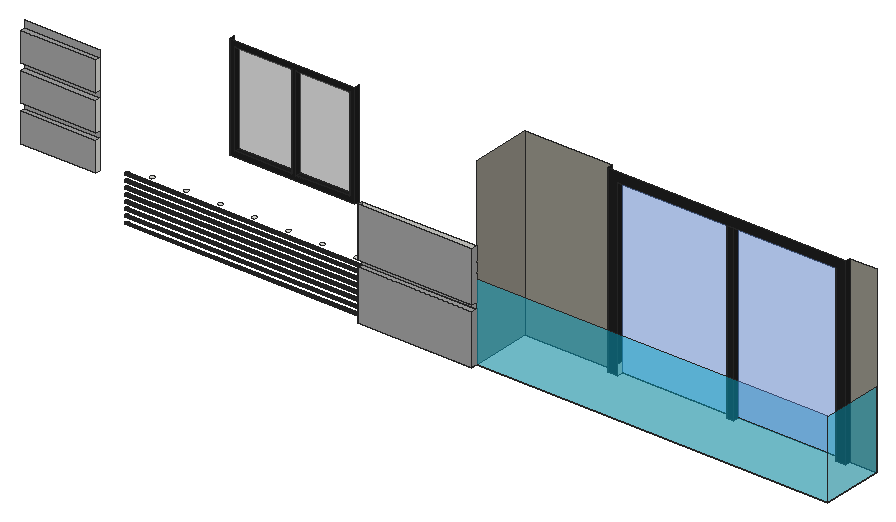
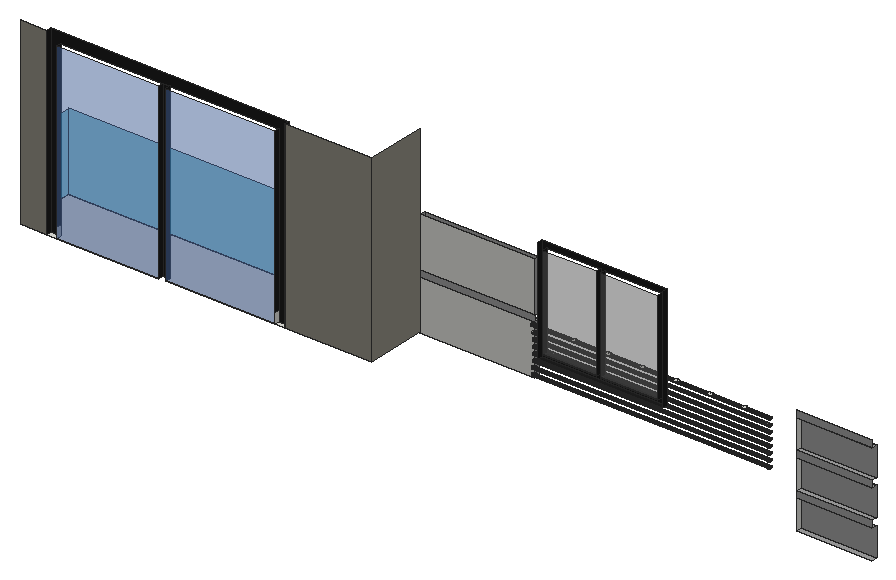
# SketchUp Ruby script. Lengths in inches.
U = 1.inch
M = Sketchup.active_model
def pt(a) = Geom::Point3d.new(a.map { |v| v * U })
def face(e, loops, mat)
  f = e.add_face(loops[0].map { |a| pt(a) })
  loops[1..].each { |l| e.add_face(l.map { |a| pt(a) }).erase! }
  f.material = f.back_material = mat if mat
  f
end
# faces: each face lists its corners as indices into pts; further lists are holes
def faces(e, pts, list, mat = nil) = list.each { |f| face(e, (f[0].is_a?(Array) ? f : [f]).map { |l| l.map { |i| pts[i] } }, mat) }
# xy, xz, yz: faces in a plane at the given z, y or x. An outline is a flat list of corners, or four numbers for a rectangle; further outlines are holes
def ring(l) = l.size == 4 ? [[l[0], l[1]], [l[2], l[1]], [l[2], l[3]], [l[0], l[3]]] : l.each_slice(2).to_a
def flat(e, list, mat, &to3) = list.each { |f| face(e, (f[0].is_a?(Array) ? f : [f]).map { |l| ring(l).map { |u, v| to3.(u, v) } }, mat) }
def xy(e, z, list, mat = nil) = flat(e, list, mat) { |x, y| [x, y, z] }
def xz(e, y, list, mat = nil) = flat(e, list, mat) { |x, z| [x, y, z] }
def yz(e, x, list, mat = nil) = flat(e, list, mat) { |y, z| [x, y, z] }
def lines(e, pts, list) = list.each { |a, b| e.add_line(pt(pts[a]), pt(pts[b])) }
# prism: a flat outline (further loops are holes) pulled along v
def prism(e, loops, v, mat = nil)
  f = face(e, loops, mat); d = Geom::Vector3d.new(v.map { |x| x * U })
  f.pushpull(f.normal.samedirection?(d) ? d.length : -d.length)
end
def box(e, o, s, mat = nil) = prism(e, [[o, [o[0] + s[0], o[1], o[2]], [o[0] + s[0], o[1] + s[1], o[2]], [o[0], o[1] + s[1], o[2]]]], [0, 0, s[2]], mat)
def at(x, y, z, deg = 0) = Geom::Transformation.translation(pt([x, y, z])) * Geom::Transformation.rotation(ORIGIN, Z_AXIS, deg.degrees)
def axes(o, x, y, z) = Geom::Transformation.new([*x, 0, *y, 0, *z, 0, *pt(o).to_a, 1])
def part(name) = M.definitions.add(name)
# library, detail: a bought-in or finely detailed component or shape, given as its bounding box
def library(name, o, s) = part(name).tap { |d| box(d.entities, o, s) }
def detail(e, o, s) = box(e.add_group.entities, o, s)
def put(e, d, t, mat = nil) = e.add_instance(d, t).tap { |i| i.material = mat if mat }
def group(e, t, mat = nil) = e.add_group.tap { |g| g.transformation = t; g.material = mat if mat }.entities
root = M.entities
M.materials.add("[0133_Gray]").color = [128, 128, 128]
M.materials.add("[Blacktop New]").color = [30, 30, 30]
M.materials.add("[Formica Graystone]").color = [149, 146, 135]
M.materials.add("[Marble Carrara Gold Floor Tile]").color = [225, 223, 217]
M.materials.add("[Pavers Flagstone Gray]").color = [162, 162, 162]
M.materials.add("[Translucent Glass Blue]").color = [100, 149, 237]
M.materials["[Translucent Glass Blue]"].alpha = 0.5
M.materials.add("[Translucent Glass Gray]").color = [128, 128, 128]
M.materials["[Translucent Glass Gray]"].alpha = 0.5
M.materials.add("[Translucent Glass Tinted]").color = [8, 201, 241]
M.materials["[Translucent Glass Tinted]"].alpha = 0.48
xy(root,368.26,[[0,36,45.0625,39]],"[Pavers Flagstone Gray]")
xy(root,369.12,[[229.62,0,297.58,3]],"[Pavers Flagstone Gray]")
xy(root,369.51,[[349.33,36,355.33,39],[484.79,36,490.79,39]])
xy(root,369.51,[[297.58,3,506.625,3,506.625,39,490.79,39,490.79,36,484.79,36,484.79,39,424.01,39,424.01,36,420.06,36,420.06,39,355.33,39,355.33,36,349.33,36,349.33,39,297.58,39]],"[Marble Carrara Gold Floor Tile]")
xy(root,385.625,[[0,36,45.0625,39]],"[Pavers Flagstone Gray]")
xy(root,389.7,[[0,36,45.0625,39]],"[Pavers Flagstone Gray]")
xy(root,399,[[229.62,0,297.58,3]],"[Pavers Flagstone Gray]")
xy(root,399.54,[[102.46,4.79,102.74,4.8,103.01,4.88,103.24,5.03,103.43,5.23,103.5625,5.48,103.625,5.75,103.61,6.02,103.53,6.29,103.39,6.52,103.18,6.71,102.94,6.84,102.67,6.91,102.39,6.9,102.13,6.82,101.89,6.67,101.7,6.47,101.57,6.22,101.51,5.95,101.52,5.68,101.6,5.41,101.75,5.17,101.95,4.99,102.19,4.85],[122.71,4.79,122.99,4.8,123.26,4.88,123.49,5.03,123.68,5.23,123.8125,5.48,123.875,5.75,123.86,6.02,123.78,6.29,123.64,6.52,123.43,6.71,123.19,6.84,122.92,6.91,122.64,6.9,122.38,6.82,122.14,6.67,121.95,6.47,121.82,6.22,121.76,5.95,121.77,5.68,121.85,5.41,122,5.17,122.2,4.99,122.44,4.85],[142.96,4.79,143.24,4.8,143.51,4.88,143.74,5.03,143.93,5.23,144.0625,5.48,144.125,5.75,144.11,6.02,144.03,6.29,143.89,6.52,143.68,6.71,143.44,6.84,143.17,6.91,142.89,6.9,142.63,6.82,142.39,6.67,142.2,6.47,142.07,6.22,142.01,5.95,142.02,5.68,142.1,5.41,142.25,5.17,142.45,4.99,142.69,4.85],[163.21,4.79,163.49,4.8,163.76,4.88,163.99,5.03,164.18,5.23,164.3125,5.48,164.375,5.75,164.36,6.02,164.28,6.29,164.14,6.52,163.93,6.71,163.69,6.84,163.42,6.91,163.14,6.9,162.88,6.82,162.64,6.67,162.45,6.47,162.32,6.22,162.26,5.95,162.27,5.68,162.35,5.41,162.5,5.17,162.7,4.99,162.94,4.85],[183.46,4.79,183.74,4.8,184.01,4.88,184.24,5.03,184.43,5.23,184.5625,5.48,184.625,5.75,184.61,6.02,184.53,6.29,184.39,6.52,184.18,6.71,183.94,6.84,183.67,6.91,183.39,6.9,183.13,6.82,182.89,6.67,182.7,6.47,182.57,6.22,182.51,5.95,182.52,5.68,182.6,5.41,182.75,5.17,182.95,4.99,183.19,4.85],
  [203.71,4.79,203.99,4.8,204.26,4.88,204.49,5.03,204.68,5.23,204.8125,5.48,204.875,5.75,204.86,6.02,204.78,6.29,204.64,6.52,204.43,6.71,204.19,6.84,203.92,6.91,203.64,6.9,203.38,6.82,203.14,6.67,202.95,6.47,202.82,6.22,202.76,5.95,202.77,5.68,202.85,5.41,203,5.17,203.2,4.99,203.44,4.85],[223.96,4.79,224.24,4.8,224.51,4.88,224.74,5.03,224.93,5.23,225.0625,5.48,225.125,5.75,225.11,6.02,225.03,6.29,224.89,6.52,224.68,6.71,224.44,6.84,224.17,6.91,223.89,6.9,223.63,6.82,223.39,6.67,223.2,6.47,223.07,6.22,223.01,5.95,223.02,5.68,223.1,5.41,223.25,5.17,223.45,4.99,223.69,4.85]])
xy(root,402.62,[[229.62,0,297.58,3]],"[Pavers Flagstone Gray]")
xy(root,405.86,[[124.42,36,198.67,39]],"[Blacktop New]")
xy(root,407.0625,[[0,36,45.0625,39]],"[Pavers Flagstone Gray]")
xy(root,408.86,[[127.42,36,161.55,39],[163.99,36,195.67,39]],"[Blacktop New]")
xy(root,411.14,[[0,36,45.0625,39]],"[Pavers Flagstone Gray]")
xy(root,428.5,[[0,36,45.0625,39]],"[Pavers Flagstone Gray]")
xz(root,0,[[229.62,369.12,297.58,399],[229.62,402.62,297.58,432.5]],"[Pavers Flagstone Gray]")
xz(root,3,[[229.62,369.12,297.58,399],[229.62,402.62,297.58,432.5]])
xz(root,3,[[229.62,399,297.58,402.62]],"[Pavers Flagstone Gray]")
xz(root,3,[[297.58,369.51,506.625,415.41]],"[Translucent Glass Tinted]")
xz(root,36,[[349.33,369.51,355.33,369.51,355.33,472.125,484.79,472.125,484.79,369.51,490.79,369.51,490.79,478.125,349.33,478.125],[420.06,369.51,424.01,472.125],[[124.42,405.86,198.67,467.74],[127.42,408.86,161.55,464.74],[163.99,408.86,195.67,464.74]]],"[Blacktop New]")
xz(root,36,[[0,368.26,45.0625,385.625],[0,389.7,45.0625,407.0625],[0,411.14,45.0625,428.5]],"[Pavers Flagstone Gray]")
xz(root,39,[[297.58,369.51,349.33,478.125],[490.79,369.51,506.625,478.125]],"[Formica Graystone]")
xz(root,39,[[0,385.625,45.0625,389.7],[0,407.0625,45.0625,411.14],[0,428.5,45.0625,432.57]],"[Pavers Flagstone Gray]")
xz(root,39,[[355.33,369.51,420.06,472.125],[424.01,369.51,484.79,472.125]],"[Translucent Glass Blue]")
xz(root,39,[[127.42,408.86,161.55,464.74],[163.99,408.86,195.67,464.74]],"[Translucent Glass Gray]")
yz(root,45.0625,[[36,368.26,39,385.625],[36,389.7,39,407.0625],[36,411.14,39,428.5]])
yz(root,124.42,[[36,405.86,39,467.74]],"[Blacktop New]")
yz(root,127.42,[[36,408.86,39,464.74]],"[Blacktop New]")
yz(root,161.55,[[36,408.86,39,464.74]],"[Blacktop New]")
yz(root,163.99,[[36,408.86,39,464.74]],"[Blacktop New]")
yz(root,195.67,[[36,408.86,39,464.74]],"[Blacktop New]")
yz(root,198.67,[[36,405.86,39,467.74]],"[Blacktop New]")
yz(root,229.62,[[0,369.12,3,399],[0,402.62,3,432.5]],"[Pavers Flagstone Gray]")
yz(root,229.85,[[3.75,393.11,3.93,393.13,4.1,393.2,4.24,393.31,4.35,393.45,4.42,393.61,4.44,393.79,4.42,393.97,4.35,394.14,4.24,394.28,4.1,394.39,3.93,394.46,3.75,394.48,3.57,394.46,3.41,394.39,3.27,394.28,3.16,394.14,3.09,393.97,3.06,393.79,3.09,393.61,3.16,393.45,3.27,393.31,3.41,393.2,3.57,393.13]])
yz(root,230.1,[[3.75,370.61,3.93,370.63,4.1,370.7,4.24,370.81,4.35,370.95,4.42,371.11,4.44,371.29,4.42,371.47,4.35,371.64,4.24,371.78,4.1,371.89,3.93,371.96,3.75,371.98,3.57,371.96,3.41,371.89,3.27,371.78,3.16,371.64,3.09,371.47,3.06,371.29,3.09,371.11,3.16,370.95,3.27,370.81,3.41,370.7,3.57,370.63]])
yz(root,230.16,[[3.75,374.36,3.93,374.38,4.1,374.45,4.24,374.56,4.35,374.7,4.42,374.86,4.44,375.04,4.42,375.22,4.35,375.39,4.24,375.53,4.1,375.64,3.93,375.71,3.75,375.73,3.57,375.71,3.41,375.64,3.27,375.53,3.16,375.39,3.09,375.22,3.06,375.04,3.09,374.86,3.16,374.7,3.27,374.56,3.41,374.45,3.57,374.38]])
yz(root,230.66,[[3.75,396.86,3.93,396.88,4.1,396.95,4.24,397.06,4.35,397.2,4.42,397.36,4.44,397.54,4.42,397.72,4.35,397.89,4.24,398.03,4.1,398.14,3.93,398.21,3.75,398.23,3.57,398.21,3.41,398.14,3.27,398.03,3.16,397.89,3.09,397.72,3.06,397.54,3.09,397.36,3.16,397.2,3.27,397.06,3.41,396.95,3.57,396.88]])
yz(root,297.58,[[0,369.12,3,369.51]])
yz(root,297.58,[[3,369.51,39,478.125]],"[Formica Graystone]")
yz(root,297.58,[[0,369.51,3,399],[0,402.62,3,432.5]],"[Pavers Flagstone Gray]")
yz(root,349.33,[[36,369.51,39,478.125]],"[Blacktop New]")
yz(root,355.33,[[36,369.51,39,375.51]])
yz(root,355.33,[[36,375.51,39,472.125]],"[Blacktop New]")
yz(root,420.06,[[36,369.51,39,472.125]],"[Blacktop New]")
yz(root,424.01,[[36,369.51,39,472.125]],"[Blacktop New]")
yz(root,484.79,[[36,369.51,39,375.51]])
yz(root,484.79,[[36,375.51,39,472.125]],"[Blacktop New]")
yz(root,490.79,[[36,369.51,39,478.125]],"[Blacktop New]")
yz(root,506.625,[[3,369.51,39,415.33]],"[Translucent Glass Tinted]")
p = [[88.53,3.41,370.7],[88.53,3.57,370.63],[230.1,3.57,370.63],[230.1,3.41,370.7],[88.53,3.75,370.61],[230.1,3.75,370.61],
  [88.53,3.93,370.63],[230.1,3.93,370.63],[88.53,4.1,370.7],[230.1,4.1,370.7],[88.53,3.27,370.81],[230.1,3.27,370.81],
  [88.53,4.24,370.81],[230.1,4.24,370.81],[88.53,3.16,370.95],[230.1,3.16,370.95],[88.53,4.35,370.95],[230.1,4.35,370.95],
  [88.53,3.09,371.11],[230.1,3.09,371.11],[88.53,4.42,371.11],[230.1,4.42,371.11],[88.53,3.06,371.29],[230.1,3.06,371.29],
  [88.53,4.44,371.29],[230.1,4.44,371.29],[88.53,3.09,371.47],[230.1,3.09,371.47],[88.53,4.42,371.47],[230.1,4.42,371.47],
  [88.53,3.16,371.64],[230.1,3.16,371.64],[88.53,4.35,371.64],[230.1,4.35,371.64],[88.53,3.27,371.78],[230.1,3.27,371.78],
  [88.53,4.24,371.78],[230.1,4.24,371.78],[88.53,3.41,371.89],[230.1,3.41,371.89],[88.53,4.1,371.89],[230.1,4.1,371.89],
  [88.53,3.57,371.96],[230.1,3.57,371.96],[88.53,3.93,371.96],[230.1,3.93,371.96],[88.53,3.75,371.98],[230.1,3.75,371.98],
  [88.53,3.27,374.56],[88.53,3.41,374.45],[230.16,3.41,374.45],[230.16,3.27,374.56],[88.53,3.57,374.38],[230.16,3.57,374.38],
  [88.53,3.75,374.36],[230.16,3.75,374.36],[88.53,3.93,374.38],[230.16,3.93,374.38],[88.53,4.1,374.45],[230.16,4.1,374.45],
  [88.53,4.24,374.56],[230.16,4.24,374.56],[88.53,3.16,374.7],[230.16,3.16,374.7],[88.53,4.35,374.7],[230.16,4.35,374.7],
  [88.53,3.09,374.86],[230.16,3.09,374.86],[88.53,4.42,374.86],[230.16,4.42,374.86],[88.53,3.06,375.04],[230.16,3.06,375.04],
  [88.53,4.44,375.04],[230.16,4.44,375.04],[88.53,3.09,375.22],[230.16,3.09,375.22],[88.53,4.42,375.22],[230.16,4.42,375.22],
  [88.53,3.16,375.39],[230.16,3.16,375.39],[88.53,4.35,375.39],[230.16,4.35,375.39],[88.53,3.27,375.53],[230.16,3.27,375.53],
  [88.53,4.24,375.53],[230.16,4.24,375.53],[88.53,3.41,375.64],[230.16,3.41,375.64],[88.53,4.1,375.64],[230.16,4.1,375.64],
  [88.53,3.57,375.71],[230.16,3.57,375.71],[88.53,3.93,375.71],[230.16,3.93,375.71],[88.53,3.75,375.73],[230.16,3.75,375.73],
  [88.53,3.41,378.2],[88.53,3.57,378.13],[229.62,3.57,378.13],[229.62,3.41,378.2],[88.53,3.75,378.11],[229.62,3.75,378.11],
  [88.53,3.93,378.13],[229.62,3.93,378.13],[88.53,4.1,378.2],[229.62,4.1,378.2],[88.53,3.27,378.31],[229.62,3.27,378.31],
  [88.53,4.24,378.31],[229.62,4.24,378.31],[88.53,3.16,378.45],[229.62,3.16,378.45],[88.53,4.35,378.45],[229.62,4.35,378.45],
  [88.53,3.09,378.61],[229.62,3.09,378.61],[88.53,4.42,378.61],[229.62,4.42,378.61],[88.53,3.06,378.79],[229.62,3.06,378.79],
  [88.53,4.44,378.79],[229.62,4.44,378.79],[88.53,3.09,378.97],[229.62,3.09,378.97],[88.53,4.42,378.97],[229.62,4.42,378.97],
  [88.53,3.16,379.14],[229.62,3.16,379.14],[88.53,4.35,379.14],[229.62,4.35,379.14],[88.53,3.27,379.28],[229.62,3.27,379.28],
  [88.53,4.24,379.28],[229.62,4.24,379.28],[88.53,3.41,379.39],[229.62,3.41,379.39],[88.53,4.1,379.39],[229.62,4.1,379.39],
  [88.53,3.57,379.46],[229.62,3.57,379.46],[88.53,3.93,379.46],[229.62,3.93,379.46],[88.53,3.75,379.48],[229.62,3.75,379.48],
  [88.53,3.27,382.06],[88.53,3.41,381.95],[229.62,3.41,381.95],[229.62,3.27,382.06],[88.53,3.57,381.88],[229.62,3.57,381.88],
  [88.53,3.75,381.86],[229.62,3.75,381.86],[88.53,3.93,381.88],[229.62,3.93,381.88],[88.53,4.1,381.95],[229.62,4.1,381.95],
  [88.53,4.24,382.06],[229.62,4.24,382.06],[88.53,3.16,382.2],[229.62,3.16,382.2],[88.53,4.35,382.2],[229.62,4.35,382.2],
  [88.53,3.09,382.36],[229.62,3.09,382.36],[88.53,4.42,382.36],[229.62,4.42,382.36],[88.53,3.06,382.54],[229.62,3.06,382.54],
  [88.53,4.44,382.54],[229.62,4.44,382.54],[88.53,3.09,382.72],[229.62,3.09,382.72],[88.53,4.42,382.72],[229.62,4.42,382.72],
  [88.53,3.16,382.89],[229.62,3.16,382.89],[88.53,4.35,382.89],[229.62,4.35,382.89],[88.53,3.27,383.03],[229.62,3.27,383.03],
  [88.53,4.24,383.03],[229.62,4.24,383.03],[88.53,3.41,383.14],[229.62,3.41,383.14],[88.53,4.1,383.14],[229.62,4.1,383.14],
  [88.53,3.57,383.21],[229.62,3.57,383.21],[88.53,3.93,383.21],[229.62,3.93,383.21],[88.53,3.75,383.23],[229.62,3.75,383.23],
  [88.53,3.41,385.7],[88.53,3.57,385.63],[229.62,3.57,385.63],[229.62,3.41,385.7],[88.53,3.75,385.61],[229.62,3.75,385.61],
  [88.53,3.93,385.63],[229.62,3.93,385.63],[88.53,4.1,385.7],[229.62,4.1,385.7],[88.53,3.27,385.81],[229.62,3.27,385.81],
  [88.53,4.24,385.81],[229.62,4.24,385.81],[88.53,3.16,385.95],[229.62,3.16,385.95],[88.53,4.35,385.95],[229.62,4.35,385.95],
  [88.53,3.09,386.11],[229.62,3.09,386.11],[88.53,4.42,386.11],[229.62,4.42,386.11],[88.53,3.06,386.29],[229.62,3.06,386.29],
  [88.53,4.44,386.29],[229.62,4.44,386.29],[88.53,3.09,386.47],[229.62,3.09,386.47],[88.53,4.42,386.47],[229.62,4.42,386.47],
  [88.53,3.16,386.64],[229.62,3.16,386.64],[88.53,4.35,386.64],[229.62,4.35,386.64],[88.53,3.27,386.78],[229.62,3.27,386.78],
  [88.53,4.24,386.78],[229.62,4.24,386.78],[88.53,3.41,386.89],[229.62,3.41,386.89],[88.53,4.1,386.89],[229.62,4.1,386.89],
  [88.53,3.57,386.96],[229.62,3.57,386.96],[88.53,3.93,386.96],[229.62,3.93,386.96],[88.53,3.75,386.98],[229.62,3.75,386.98],
  [88.53,3.27,389.56],[88.53,3.41,389.45],[229.62,3.41,389.45],[229.62,3.27,389.56],[88.53,3.57,389.38],[229.62,3.57,389.38],
  [88.53,3.75,389.36],[229.62,3.75,389.36],[88.53,3.93,389.38],[229.62,3.93,389.38],[88.53,4.1,389.45],[229.62,4.1,389.45],
  [88.53,4.24,389.56],[229.62,4.24,389.56],[88.53,3.16,389.7],[229.62,3.16,389.7],[88.53,4.35,389.7],[229.62,4.35,389.7],
  [88.53,3.09,389.86],[229.62,3.09,389.86],[88.53,4.42,389.86],[229.62,4.42,389.86],[88.53,3.06,390.04],[229.62,3.06,390.04],
  [88.53,4.44,390.04],[229.62,4.44,390.04],[88.53,3.09,390.22],[229.62,3.09,390.22],[88.53,4.42,390.22],[229.62,4.42,390.22],
  [88.53,3.16,390.39],[229.62,3.16,390.39],[88.53,4.35,390.39],[229.62,4.35,390.39],[88.53,3.27,390.53],[229.62,3.27,390.53],
  [88.53,4.24,390.53],[229.62,4.24,390.53],[88.53,3.41,390.64],[229.62,3.41,390.64],[88.53,4.1,390.64],[229.62,4.1,390.64],
  [88.53,3.57,390.71],[229.62,3.57,390.71],[88.53,3.93,390.71],[229.62,3.93,390.71],[88.53,3.75,390.73],[229.62,3.75,390.73],
  [88.53,3.41,393.2],[88.53,3.57,393.13],[229.85,3.57,393.13],[229.85,3.41,393.2],[88.53,3.75,393.11],[229.85,3.75,393.11],
  [88.53,3.93,393.13],[229.85,3.93,393.13],[88.53,4.1,393.2],[229.85,4.1,393.2],[88.53,3.27,393.31],[229.85,3.27,393.31],
  [88.53,4.24,393.31],[229.85,4.24,393.31],[88.53,3.16,393.45],[229.85,3.16,393.45],[88.53,4.35,393.45],[229.85,4.35,393.45],
  [88.53,3.09,393.61],[229.85,3.09,393.61],[88.53,4.42,393.61],[229.85,4.42,393.61],[88.53,3.06,393.79],[229.85,3.06,393.79],
  [88.53,4.44,393.79],[229.85,4.44,393.79],[88.53,3.09,393.97],[229.85,3.09,393.97],[88.53,4.42,393.97],[229.85,4.42,393.97],
  [88.53,3.16,394.14],[229.85,3.16,394.14],[88.53,4.35,394.14],[229.85,4.35,394.14],[88.53,3.27,394.28],[229.85,3.27,394.28],
  [88.53,4.24,394.28],[229.85,4.24,394.28],[88.53,3.41,394.39],[229.85,3.41,394.39],[88.53,4.1,394.39],[229.85,4.1,394.39],
  [88.53,3.57,394.46],[229.85,3.57,394.46],[88.53,3.93,394.46],[229.85,3.93,394.46],[88.53,3.75,394.48],[229.85,3.75,394.48],
  [88.53,3.27,397.06],[88.53,3.41,396.95],[230.66,3.41,396.95],[230.66,3.27,397.06],[88.53,3.57,396.88],[230.66,3.57,396.88],
  [88.53,3.75,396.86],[230.66,3.75,396.86],[88.53,3.93,396.88],[230.66,3.93,396.88],[88.53,4.1,396.95],[230.66,4.1,396.95],
  [88.53,4.24,397.06],[230.66,4.24,397.06],[88.53,3.16,397.2],[230.66,3.16,397.2],[88.53,4.35,397.2],[230.66,4.35,397.2],
  [88.53,3.09,397.36],[230.66,3.09,397.36],[88.53,4.42,397.36],[230.66,4.42,397.36],[88.53,3.06,397.54],[230.66,3.06,397.54],
  [88.53,4.44,397.54],[230.66,4.44,397.54],[88.53,3.09,397.72],[230.66,3.09,397.72],[88.53,4.42,397.72],[230.66,4.42,397.72],
  [88.53,3.16,397.89],[230.66,3.16,397.89],[88.53,4.35,397.89],[230.66,4.35,397.89],[88.53,3.27,398.03],[230.66,3.27,398.03],
  [88.53,4.24,398.03],[230.66,4.24,398.03],[88.53,3.41,398.14],[230.66,3.41,398.14],[88.53,4.1,398.14],[230.66,4.1,398.14],
  [88.53,3.57,398.21],[230.66,3.57,398.21],[88.53,3.93,398.21],[230.66,3.93,398.21],[88.53,3.75,398.23],[230.66,3.75,398.23]]
faces(root,p,[[0,1,2,3],[1,4,5,2],[4,6,7,5],[6,8,9,7],[10,0,3,11],[8,12,13,9],[14,10,11,15],[12,16,17,13],
  [18,14,15,19],[16,20,21,17],[22,18,19,23],[20,24,25,21],[26,22,23,27],[24,28,29,25],[30,26,27,31],[28,32,33,29],
  [34,30,31,35],[32,36,37,33],[38,34,35,39],[36,40,41,37],[42,38,39,43],[40,44,45,41],[46,42,43,47],[44,46,47,45],
  [48,49,50,51],[49,52,53,50],[52,54,55,53],[54,56,57,55],[56,58,59,57],[58,60,61,59],[62,48,51,63],[60,64,65,61],
  [66,62,63,67],[64,68,69,65],[70,66,67,71],[68,72,73,69],[74,70,71,75],[72,76,77,73],[78,74,75,79],[76,80,81,77],
  [82,78,79,83],[80,84,85,81],[86,82,83,87],[84,88,89,85],[90,86,87,91],[88,92,93,89],[94,90,91,95],[92,94,95,93],
  [96,97,98,99],[97,100,101,98],[100,102,103,101],[102,104,105,103],[106,96,99,107],[104,108,109,105],[110,106,107,111],[108,112,113,109],
  [114,110,111,115],[112,116,117,113],[118,114,115,119],[116,120,121,117],[122,118,119,123],[120,124,125,121],[126,122,123,127],[124,128,129,125],
  [130,126,127,131],[128,132,133,129],[134,130,131,135],[132,136,137,133],[138,134,135,139],[136,140,141,137],[142,138,139,143],[140,142,143,141],
  [144,145,146,147],[145,148,149,146],[148,150,151,149],[150,152,153,151],[152,154,155,153],[154,156,157,155],[158,144,147,159],[156,160,161,157],
  [162,158,159,163],[160,164,165,161],[166,162,163,167],[164,168,169,165],[170,166,167,171],[168,172,173,169],[174,170,171,175],[172,176,177,173],
  [178,174,175,179],[176,180,181,177],[182,178,179,183],[180,184,185,181],[186,182,183,187],[184,188,189,185],[190,186,187,191],[188,190,191,189],
  [192,193,194,195],[193,196,197,194],[196,198,199,197],[198,200,201,199],[202,192,195,203],[200,204,205,201],[206,202,203,207],[204,208,209,205],
  [210,206,207,211],[208,212,213,209],[214,210,211,215],[212,216,217,213],[218,214,215,219],[216,220,221,217],[222,218,219,223],[220,224,225,221],
  [226,222,223,227],[224,228,229,225],[230,226,227,231],[228,232,233,229],[234,230,231,235],[232,236,237,233],[238,234,235,239],[236,238,239,237],
  [240,241,242,243],[241,244,245,242],[244,246,247,245],[246,248,249,247],[248,250,251,249],[250,252,253,251],[254,240,243,255],[252,256,257,253],
  [258,254,255,259],[256,260,261,257],[262,258,259,263],[260,264,265,261],[266,262,263,267],[264,268,269,265],[270,266,267,271],[268,272,273,269],
  [274,270,271,275],[272,276,277,273],[278,274,275,279],[276,280,281,277],[282,278,279,283],[280,284,285,281],[286,282,283,287],[284,286,287,285],
  [288,289,290,291],[289,292,293,290],[292,294,295,293],[294,296,297,295],[298,288,291,299],[296,300,301,297],[302,298,299,303],[300,304,305,301],
  [306,302,303,307],[304,308,309,305],[310,306,307,311],[308,312,313,309],[314,310,311,315],[312,316,317,313],[318,314,315,319],[316,320,321,317],
  [322,318,319,323],[320,324,325,321],[326,322,323,327],[324,328,329,325],[330,326,327,331],[328,332,333,329],[334,330,331,335],[332,334,335,333],
  [336,337,338,339],[337,340,341,338],[340,342,343,341],[342,344,345,343],[344,346,347,345],[346,348,349,347],[350,336,339,351],[348,352,353,349],
  [354,350,351,355],[352,356,357,353],[358,354,355,359],[356,360,361,357],[362,358,359,363],[360,364,365,361],[366,362,363,367],[364,368,369,365],
  [370,366,367,371],[368,372,373,369],[374,370,371,375],[372,376,377,373],[378,374,375,379],[376,380,381,377],[382,378,379,383],[380,382,383,381]],"[0133_Gray]")
